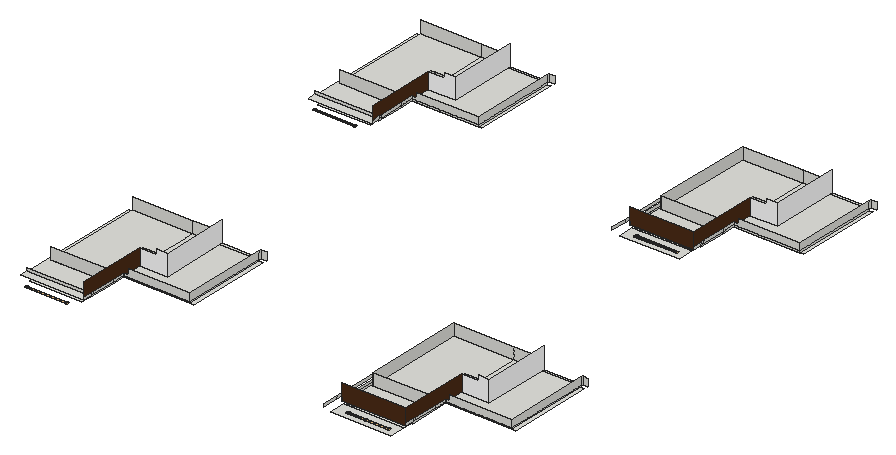
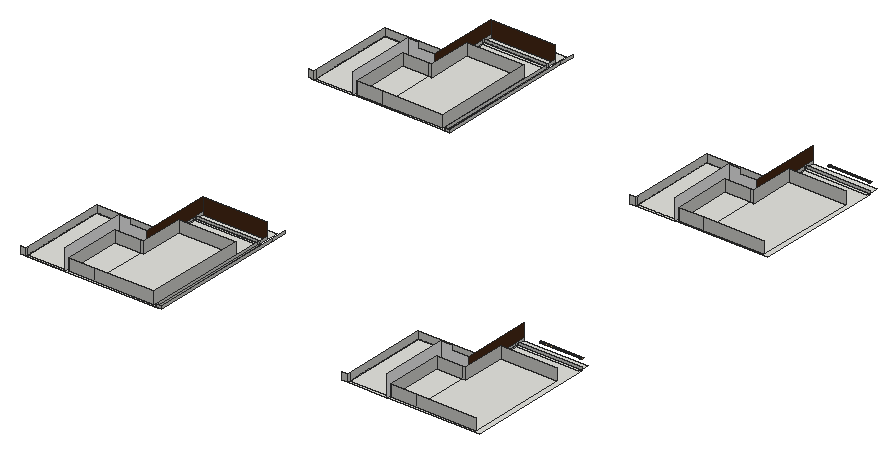
# SketchUp Ruby script. Lengths in inches.
U = 1.inch
M = Sketchup.active_model
def pt(a) = Geom::Point3d.new(a.map { |v| v * U })
def face(e, loops, mat)
  f = e.add_face(loops[0].map { |a| pt(a) })
  loops[1..].each { |l| e.add_face(l.map { |a| pt(a) }).erase! }
  f.material = f.back_material = mat if mat
  f
end
# faces: each face lists its corners as indices into pts; further lists are holes
def faces(e, pts, list, mat = nil) = list.each { |f| face(e, (f[0].is_a?(Array) ? f : [f]).map { |l| l.map { |i| pts[i] } }, mat) }
# xy, xz, yz: faces in a plane at the given z, y or x. An outline is a flat list of corners, or four numbers for a rectangle; further outlines are holes
def ring(l) = l.size == 4 ? [[l[0], l[1]], [l[2], l[1]], [l[2], l[3]], [l[0], l[3]]] : l.each_slice(2).to_a
def flat(e, list, mat, &to3) = list.each { |f| face(e, (f[0].is_a?(Array) ? f : [f]).map { |l| ring(l).map { |u, v| to3.(u, v) } }, mat) }
def xy(e, z, list, mat = nil) = flat(e, list, mat) { |x, y| [x, y, z] }
def xz(e, y, list, mat = nil) = flat(e, list, mat) { |x, z| [x, y, z] }
def yz(e, x, list, mat = nil) = flat(e, list, mat) { |y, z| [x, y, z] }
def lines(e, pts, list) = list.each { |a, b| e.add_line(pt(pts[a]), pt(pts[b])) }
# prism: a flat outline (further loops are holes) pulled along v
def prism(e, loops, v, mat = nil)
  f = face(e, loops, mat); d = Geom::Vector3d.new(v.map { |x| x * U })
  f.pushpull(f.normal.samedirection?(d) ? d.length : -d.length)
end
def box(e, o, s, mat = nil) = prism(e, [[o, [o[0] + s[0], o[1], o[2]], [o[0] + s[0], o[1] + s[1], o[2]], [o[0], o[1] + s[1], o[2]]]], [0, 0, s[2]], mat)
def at(x, y, z, deg = 0) = Geom::Transformation.translation(pt([x, y, z])) * Geom::Transformation.rotation(ORIGIN, Z_AXIS, deg.degrees)
def axes(o, x, y, z) = Geom::Transformation.new([*x, 0, *y, 0, *z, 0, *pt(o).to_a, 1])
def part(name) = M.definitions.add(name)
# library, detail: a bought-in or finely detailed component or shape, given as its bounding box
def library(name, o, s) = part(name).tap { |d| box(d.entities, o, s) }
def detail(e, o, s) = box(e.add_group.entities, o, s)
def put(e, d, t, mat = nil) = e.add_instance(d, t).tap { |i| i.material = mat if mat }
def group(e, t, mat = nil) = e.add_group.tap { |g| g.transformation = t; g.material = mat if mat }.entities
root = M.entities
M.materials.add("[Color M00]").color = [255, 255, 255]
M.materials.add("[Wood Veneer 01]").color = [76, 44, 23]
c1 = library("Group\#25",[-0.5,-0.5,-0.05],[119,6.375,0.22])
xy(root,257.1875,[[[2977.35,592.75,3143.91,636.6875],[3008.92,609.37,3009.62,609.46,3010.27,609.73,3010.82,610.15,3011.25,610.71,3011.52,611.36,3011.61,612.06,3011.52,612.75,3011.25,613.4,3010.82,613.96,3010.27,614.38,3009.62,614.65,3008.92,614.74,3008.23,614.65,3007.58,614.38,3007.02,613.96,3006.6,613.4,3006.33,612.75,3006.24,612.06,3006.33,611.36,3006.6,610.71,3007.02,610.15,3007.58,609.73,3008.23,609.46],[3056.92,609.37,3057.62,609.46,3058.27,609.73,3058.82,610.15,3059.25,610.71,3059.52,611.36,3059.61,612.06,3059.52,612.75,3059.25,613.4,3058.82,613.96,3058.27,614.38,3057.62,614.65,3056.92,614.74,3056.23,614.65,3055.58,614.38,3055.02,613.96,3054.6,613.4,3054.33,612.75,3054.24,612.06,3054.33,611.36,3054.6,610.71,3055.02,610.15,3055.58,609.73,3056.23,609.46],[3121.55,609.37,3122.24,609.46,3122.89,609.73,3123.45,610.15,3123.875,610.71,3124.14,611.36,3124.24,612.06,3124.14,612.75,3123.875,613.4,3123.45,613.96,3122.89,614.38,3122.24,614.65,3121.55,614.74,3120.85,614.65,3120.2,614.38,3119.65,613.96,3119.22,613.4,3118.95,612.75,3118.86,612.06,3118.95,611.36,3119.22,610.71,3119.65,610.15,3120.2,609.73,3120.85,609.46]],[2106.51,636.6875,2251.32,660.21],[2986.73,636.6875,2999.1,660.21],[2999.1,636.6875,3143.91,660.21],[[2977.35,1592.1,3143.91,1636.04],[3008.92,1608.72,3009.62,1608.8125,3010.27,1609.08,3010.82,1609.51,3011.25,1610.07,3011.52,1610.71,3011.61,1611.41,3011.52,1612.11,3011.25,1612.75,3010.82,1613.3125,3010.27,1613.74,3009.62,1614.01,3008.92,1614.1,3008.23,1614.01,3007.58,1613.74,3007.02,1613.3125,3006.6,1612.75,3006.33,1612.11,3006.24,1611.41,3006.33,1610.71,3006.6,1610.07,3007.02,1609.51,3007.58,1609.08,3008.23,1608.8125],[3056.92,1608.72,3057.62,1608.8125,3058.27,1609.08,3058.82,1609.51,3059.25,1610.07,3059.52,1610.71,3059.61,1611.41,3059.52,1612.11,3059.25,1612.75,3058.82,1613.3125,3058.27,1613.74,3057.62,1614.01,3056.92,1614.1,3056.23,1614.01,3055.58,1613.74,3055.02,1613.3125,3054.6,1612.75,3054.33,1612.11,3054.24,1611.41,3054.33,1610.71,3054.6,1610.07,3055.02,1609.51,3055.58,1609.08,3056.23,1608.8125],[3121.55,1608.72,3122.24,1608.8125,3122.89,1609.08,3123.45,1609.51,3123.875,1610.07,3124.14,1610.71,3124.24,1611.41,3124.14,1612.11,3123.875,1612.75,3123.45,1613.3125,3122.89,1613.74,3122.24,1614.01,3121.55,1614.1,3120.85,1614.01,3120.2,1613.74,3119.65,1613.3125,3119.22,1612.75,3118.95,1612.11,3118.86,1611.41,3118.95,1610.71,3119.22,1610.07,3119.65,1609.51,3120.2,1609.08,3120.85,1608.8125]],
  [2106.51,1636.04,2251.32,1659.57],[2986.73,1636.04,2999.1,1659.57],[2999.1,1636.04,3143.91,1659.57]])
xy(root,259.3125,[[2079.65,660.21,2079.65,1012.63,2440.84,1012.63,2440.84,774.3125,2256.86,774.3125,2256.86,660.21],[2972.24,660.21,2972.24,1012.63,3333.43,1012.63,3333.43,774.3125,3149.44,774.3125,3149.44,660.21],[2440.84,774.3125,2450.84,1012.63],[3333.43,774.3125,3343.43,1012.63],[2079.65,1659.57,2079.65,2011.98,2440.84,2011.98,2440.84,1773.67,2256.86,1773.67,2256.86,1659.57],
  [2972.24,1659.57,2972.24,2011.98,3333.43,2011.98,3333.43,1773.67,3149.44,1773.67,3149.44,1659.57],[2440.84,1773.67,2450.84,2011.98],[3333.43,1773.67,3343.43,2011.98]])
xy(root,262.875,[[2079.65,636.86,2256.86,660.21],[2972.24,636.86,3149.44,660.21],[2079.65,660.21,2256.86,668.18],[2972.24,660.21,3149.44,668.18],[2089.96,731.45,2247.33,731.45,2247.33,852.1875,2256.86,852.1875,2256.86,1012.63,2089.96,1012.63],
  [2982.55,731.45,3139.92,731.45,3139.92,852.1875,3149.44,852.1875,3149.44,1012.63,2982.55,1012.63],[2256.86,774.3125,2440.84,774.3125,2440.84,1012.63,2333.29,1012.63,2333.29,829.8125,2256.86,829.8125],[3149.44,774.3125,3333.43,774.3125,3333.43,1012.63,3225.88,1012.63,3225.88,829.8125,3149.44,829.8125],[2256.86,852.1875,2327.29,1012.63],[3149.44,852.1875,3219.88,1012.63],
  [2333.29,1012.63,2440.84,1019],[3225.88,1012.63,3333.43,1019],[2079.65,1636.22,2256.86,1659.57],[2972.24,1636.22,3149.44,1659.57],[2079.65,1659.57,2256.86,1667.53],
  [2972.24,1659.57,3149.44,1667.53],[2089.96,1730.8,2247.33,1730.8,2247.33,1851.54,2256.86,1851.54,2256.86,2011.98,2089.96,2011.98],[2982.55,1730.8,3139.92,1730.8,3139.92,1851.54,3149.44,1851.54,3149.44,2011.98,2982.55,2011.98],[2256.86,1773.67,2440.84,1773.67,2440.84,2011.98,2333.29,2011.98,2333.29,1829.17,2256.86,1829.17],[3149.44,1773.67,3333.43,1773.67,3333.43,2011.98,3225.88,2011.98,3225.88,1829.17,3149.44,1829.17],
  [2256.86,1851.54,2327.29,2011.98],[3149.44,1851.54,3219.88,2011.98],[2333.29,2011.98,2440.84,2018.36],[3225.88,2011.98,3333.43,2018.36]])
xz(root,636.86,[[2972.24,262.875,3149.44,307.5]],"[Wood Veneer 01]")
xz(root,660.21,[[2972.24,259.3125,3149.44,262.875],[2079.65,262.875,2256.86,270.375],[2972.24,262.875,3149.44,270.375]])
xz(root,731.45,[[2089.96,262.875,2247.33,295.8125],[2982.55,262.875,3139.92,295.8125]])
xz(root,774.3125,[[2256.86,259.3125,2440.84,262.875],[3149.44,259.3125,3333.43,262.875],[2256.86,262.875,2256.86,270.375,2269.48,270.375,2269.48,283.9375,2440.84,283.9375,2440.84,262.875],[3149.44,262.875,3149.44,270.375,3162.07,270.375,3162.07,283.9375,3333.43,283.9375,3333.43,262.875]])
xz(root,829.8125,[[2256.86,262.875,2333.29,262.875,2333.29,320.75,2303.29,320.75,2303.29,307.5,2256.86,307.5],[3149.44,262.875,3225.88,262.875,3225.88,320.75,3195.88,320.75,3195.88,307.5,3149.44,307.5]],"[Color M00]")
xz(root,852.1875,[[2247.33,262.875,2256.86,295.8125],[2256.86,262.875,2327.29,295.8125],[3139.92,262.875,3149.44,295.8125],[3149.44,262.875,3219.88,295.8125]])
xz(root,1012.63,[[2089.96,262.875,2256.86,295.8125],[2256.86,262.875,2327.29,295.8125],[2982.55,262.875,3149.44,295.8125],[3149.44,262.875,3219.88,295.8125]])
xz(root,1019,[[2440.84,262.875,2456.54,283.9375],[2957.51,262.875,2972.24,270.375],[3333.43,262.875,3349.13,283.9375]])
xz(root,1636.22,[[2972.24,262.875,3149.44,307.5]],"[Wood Veneer 01]")
xz(root,1659.57,[[2972.24,259.3125,3149.44,262.875],[2079.65,262.875,2256.86,270.375],[2972.24,262.875,3149.44,270.375]])
xz(root,1730.8,[[2089.96,262.875,2247.33,295.8125],[2982.55,262.875,3139.92,295.8125]])
xz(root,1773.67,[[2256.86,259.3125,2440.84,262.875],[3149.44,259.3125,3333.43,262.875],[2256.86,262.875,2256.86,270.375,2269.48,270.375,2269.48,283.9375,2440.84,283.9375,2440.84,262.875],[3149.44,262.875,3149.44,270.375,3162.07,270.375,3162.07,283.9375,3333.43,283.9375,3333.43,262.875]])
xz(root,1829.17,[[2256.86,262.875,2333.29,262.875,2333.29,320.75,2303.29,320.75,2303.29,307.5,2256.86,307.5],[3149.44,262.875,3225.88,262.875,3225.88,320.75,3195.88,320.75,3195.88,307.5,3149.44,307.5]],"[Color M00]")
xz(root,1851.54,[[2247.33,262.875,2256.86,295.8125],[2256.86,262.875,2327.29,295.8125],[3139.92,262.875,3149.44,295.8125],[3149.44,262.875,3219.88,295.8125]])
xz(root,2011.98,[[2089.96,262.875,2256.86,295.8125],[2256.86,262.875,2327.29,295.8125],[2982.55,262.875,3149.44,295.8125],[3149.44,262.875,3219.88,295.8125]])
xz(root,2018.36,[[2440.84,262.875,2456.54,283.9375],[2957.51,262.875,2972.24,270.375],[3333.43,262.875,3349.13,283.9375]])
yz(root,2247.33,[[731.45,262.875,852.1875,295.8125],[1730.8,262.875,1851.54,295.8125]])
yz(root,2256.86,[[660.21,259.3125,735.75,262.875],[735.75,259.3125,774.3125,262.875],[1659.57,259.3125,1735.1,262.875],[1735.1,259.3125,1773.67,262.875],[636.86,262.875,660.21,270.375],
  [660.21,262.875,668.18,270.375],[668.18,262.875,735.75,270.375],[735.75,262.875,774.3125,270.375],[1636.22,262.875,1659.57,270.375],[1659.57,262.875,1667.53,270.375],
  [1667.53,262.875,1735.1,270.375],[1735.1,262.875,1773.67,270.375]])
yz(root,2256.86,[[774.3125,262.875,829.8125,262.875,829.8125,307.5,636.86,307.5,636.86,270.375,774.3125,270.375],[1773.67,262.875,1829.17,262.875,1829.17,307.5,1636.22,307.5,1636.22,270.375,1773.67,270.375]],"[Wood Veneer 01]")
yz(root,2327.29,[[852.1875,262.875,1012.63,295.8125],[1851.54,262.875,2011.98,295.8125]])
yz(root,2333.29,[[829.8125,262.875,1019,320.75],[1829.17,262.875,2018.36,320.75]],"[Color M00]")
yz(root,2440.84,[[774.3125,259.3125,1012.63,262.875],[1773.67,259.3125,2011.98,262.875],[774.3125,262.875,1012.63,283.9375],[1012.63,262.875,1019,283.9375],[1773.67,262.875,2011.98,283.9375],
  [2011.98,262.875,2018.36,283.9375]])
yz(root,2957.51,[[592.75,262.875,636.6875,270.375],[636.6875,262.875,1019,270.375],[1592.1,262.875,1636.04,270.375],[1636.04,262.875,2018.36,270.375]])
yz(root,2972.24,[[660.21,259.3125,1012.63,262.875],[1659.57,259.3125,2011.98,262.875],[636.86,262.875,660.21,270.375],[660.21,262.875,668.18,270.375],[668.18,262.875,1012.63,270.375],
  [1012.63,262.875,1019,270.375],[1636.22,262.875,1659.57,270.375],[1659.57,262.875,1667.53,270.375],[1667.53,262.875,2011.98,270.375],[2011.98,262.875,2018.36,270.375]])
yz(root,2982.55,[[731.45,262.875,1012.63,295.8125],[1730.8,262.875,2011.98,295.8125]])
yz(root,3139.92,[[731.45,262.875,852.1875,295.8125],[1730.8,262.875,1851.54,295.8125]])
yz(root,3149.44,[[660.21,259.3125,735.75,262.875],[735.75,259.3125,774.3125,262.875],[1659.57,259.3125,1735.1,262.875],[1735.1,259.3125,1773.67,262.875],[636.86,262.875,660.21,270.375],
  [660.21,262.875,668.18,270.375],[668.18,262.875,735.75,270.375],[735.75,262.875,774.3125,270.375],[1636.22,262.875,1659.57,270.375],[1659.57,262.875,1667.53,270.375],
  [1667.53,262.875,1735.1,270.375],[1735.1,262.875,1773.67,270.375]])
yz(root,3149.44,[[774.3125,262.875,829.8125,262.875,829.8125,307.5,636.86,307.5,636.86,270.375,774.3125,270.375],[1773.67,262.875,1829.17,262.875,1829.17,307.5,1636.22,307.5,1636.22,270.375,1773.67,270.375]],"[Wood Veneer 01]")
yz(root,3219.88,[[852.1875,262.875,1012.63,295.8125],[1851.54,262.875,2011.98,295.8125]])
yz(root,3225.88,[[829.8125,262.875,1019,320.75],[1829.17,262.875,2018.36,320.75]],"[Color M00]")
yz(root,3333.43,[[774.3125,259.3125,1012.63,262.875],[1773.67,259.3125,2011.98,262.875],[774.3125,262.875,1012.63,283.9375],[1012.63,262.875,1019,283.9375],[1773.67,262.875,2011.98,283.9375],
  [2011.98,262.875,2018.36,283.9375]])
p = [[2228.96,609.37,257.1875],[2228.26,609.46,257.1875],[2228.26,609.46,257.8125],[2228.96,609.37,257.8125],[2229.65,609.46,257.1875],[2229.65,609.46,257.8125],
  [3008.92,609.37,257.1875],[3008.23,609.46,257.1875],[3008.23,609.46,257.6875],[3008.92,609.37,257.6875],[3009.62,609.46,257.1875],[3009.62,609.46,257.6875],
  [3056.92,609.37,257.1875],[3056.23,609.46,257.1875],[3056.23,609.46,257.8125],[3056.92,609.37,257.8125],[3057.62,609.46,257.1875],[3057.62,609.46,257.8125],
  [3121.55,609.37,257.1875],[3120.85,609.46,257.1875],[3120.85,609.46,257.8125],[3121.55,609.37,257.8125],[3122.24,609.46,257.1875],[3122.24,609.46,257.8125],
  [2227.61,609.73,257.1875],[2227.61,609.73,257.8125],[2230.3,609.73,257.1875],[2230.3,609.73,257.8125],[3007.58,609.73,257.1875],[3007.58,609.73,257.6875],
  [3010.27,609.73,257.1875],[3010.27,609.73,257.6875],[3055.58,609.73,257.1875],[3055.58,609.73,257.8125],[3058.27,609.73,257.1875],[3058.27,609.73,257.8125],
  [3120.2,609.73,257.1875],[3120.2,609.73,257.8125],[3122.89,609.73,257.1875],[3122.89,609.73,257.8125],[2227.06,610.15,257.1875],[2227.06,610.15,257.8125],
  [2230.86,610.15,257.1875],[2230.86,610.15,257.8125],[3007.02,610.15,257.1875],[3007.02,610.15,257.6875],[3010.82,610.15,257.1875],[3010.82,610.15,257.6875],
  [3055.02,610.15,257.1875],[3055.02,610.15,257.8125],[3058.82,610.15,257.1875],[3058.82,610.15,257.8125],[3119.65,610.15,257.1875],[3119.65,610.15,257.8125],
  [3123.45,610.15,257.1875],[3123.45,610.15,257.8125],[2226.63,610.71,257.1875],[2226.63,610.71,257.8125],[2231.29,610.71,257.1875],[2231.29,610.71,257.8125],
  [3006.6,610.71,257.1875],[3006.6,610.71,257.6875],[3011.25,610.71,257.1875],[3011.25,610.71,257.6875],[3054.6,610.71,257.1875],[3054.6,610.71,257.8125],
  [3059.25,610.71,257.1875],[3059.25,610.71,257.8125],[3119.22,610.71,257.1875],[3119.22,610.71,257.8125],[3123.875,610.71,257.1875],[3123.875,610.71,257.8125],
  [2226.36,611.36,257.1875],[2226.36,611.36,257.8125],[2231.55,611.36,257.1875],[2231.55,611.36,257.8125],[3006.33,611.36,257.1875],[3006.33,611.36,257.6875],
  [3011.52,611.36,257.1875],[3011.52,611.36,257.6875],[3054.33,611.36,257.1875],[3054.33,611.36,257.8125],[3059.52,611.36,257.1875],[3059.52,611.36,257.8125],
  [3118.95,611.36,257.1875],[3118.95,611.36,257.8125],[3124.14,611.36,257.1875],[3124.14,611.36,257.8125],[2226.27,612.06,257.1875],[2226.27,612.06,257.8125],
  [2231.65,612.06,257.1875],[2231.65,612.06,257.8125],[3006.24,612.06,257.1875],[3006.24,612.06,257.6875],[3011.61,612.06,257.1875],[3011.61,612.06,257.6875],
  [3054.24,612.06,257.1875],[3054.24,612.06,257.8125],[3059.61,612.06,257.1875],[3059.61,612.06,257.8125],[3118.86,612.06,257.1875],[3118.86,612.06,257.8125],
  [3124.24,612.06,257.1875],[3124.24,612.06,257.8125],[2226.36,612.75,257.1875],[2226.36,612.75,257.8125],[2231.55,612.75,257.1875],[2231.55,612.75,257.8125],
  [3006.33,612.75,257.1875],[3006.33,612.75,257.6875],[3011.52,612.75,257.1875],[3011.52,612.75,257.6875],[3054.33,612.75,257.1875],[3054.33,612.75,257.8125],
  [3059.52,612.75,257.1875],[3059.52,612.75,257.8125],[3118.95,612.75,257.1875],[3118.95,612.75,257.8125],[3124.14,612.75,257.1875],[3124.14,612.75,257.8125],
  [2226.63,613.4,257.1875],[2226.63,613.4,257.8125],[2231.29,613.4,257.1875],[2231.29,613.4,257.8125],[3006.6,613.4,257.1875],[3006.6,613.4,257.6875],
  [3011.25,613.4,257.1875],[3011.25,613.4,257.6875],[3054.6,613.4,257.1875],[3054.6,613.4,257.8125],[3059.25,613.4,257.1875],[3059.25,613.4,257.8125],
  [3119.22,613.4,257.1875],[3119.22,613.4,257.8125],[3123.875,613.4,257.1875],[3123.875,613.4,257.8125],[2227.06,613.96,257.1875],[2227.06,613.96,257.8125],
  [2230.86,613.96,257.1875],[2230.86,613.96,257.8125],[3007.02,613.96,257.1875],[3007.02,613.96,257.6875],[3010.82,613.96,257.1875],[3010.82,613.96,257.6875],
  [3055.02,613.96,257.1875],[3055.02,613.96,257.8125],[3058.82,613.96,257.1875],[3058.82,613.96,257.8125],[3119.65,613.96,257.1875],[3119.65,613.96,257.8125],
  [3123.45,613.96,257.1875],[3123.45,613.96,257.8125],[2227.61,614.38,257.1875],[2227.61,614.38,257.8125],[2230.3,614.38,257.1875],[2230.3,614.38,257.8125],
  [3007.58,614.38,257.1875],[3007.58,614.38,257.6875],[3010.27,614.38,257.1875],[3010.27,614.38,257.6875],[3055.58,614.38,257.1875],[3055.58,614.38,257.8125],
  [3058.27,614.38,257.1875],[3058.27,614.38,257.8125],[3120.2,614.38,257.1875],[3120.2,614.38,257.8125],[3122.89,614.38,257.1875],[3122.89,614.38,257.8125],
  [2228.26,614.65,257.1875],[2228.26,614.65,257.8125],[2229.65,614.65,257.1875],[2229.65,614.65,257.8125],[3008.23,614.65,257.1875],[3008.23,614.65,257.6875],
  [3009.62,614.65,257.1875],[3009.62,614.65,257.6875],[3056.23,614.65,257.1875],[3056.23,614.65,257.8125],[3057.62,614.65,257.1875],[3057.62,614.65,257.8125],
  [3120.85,614.65,257.1875],[3120.85,614.65,257.8125],[3122.24,614.65,257.1875],[3122.24,614.65,257.8125],[2228.96,614.74,257.1875],[2228.96,614.74,257.8125],
  [3008.92,614.74,257.1875],[3008.92,614.74,257.6875],[3056.92,614.74,257.1875],[3056.92,614.74,257.8125],[3121.55,614.74,257.1875],[3121.55,614.74,257.8125],
  [2228.96,1608.72,257.1875],[2228.26,1608.8125,257.1875],[2228.26,1608.8125,257.8125],[2228.96,1608.72,257.8125],[2229.65,1608.8125,257.1875],[2229.65,1608.8125,257.8125],
  [3008.92,1608.72,257.1875],[3008.23,1608.8125,257.1875],[3008.23,1608.8125,257.6875],[3008.92,1608.72,257.6875],[3009.62,1608.8125,257.1875],[3009.62,1608.8125,257.6875],
  [3056.92,1608.72,257.1875],[3056.23,1608.8125,257.1875],[3056.23,1608.8125,257.8125],[3056.92,1608.72,257.8125],[3057.62,1608.8125,257.1875],[3057.62,1608.8125,257.8125],
  [3121.55,1608.72,257.1875],[3120.85,1608.8125,257.1875],[3120.85,1608.8125,257.8125],[3121.55,1608.72,257.8125],[3122.24,1608.8125,257.1875],[3122.24,1608.8125,257.8125],
  [2227.61,1609.08,257.1875],[2227.61,1609.08,257.8125],[2230.3,1609.08,257.1875],[2230.3,1609.08,257.8125],[3007.58,1609.08,257.1875],[3007.58,1609.08,257.6875],
  [3010.27,1609.08,257.1875],[3010.27,1609.08,257.6875],[3055.58,1609.08,257.1875],[3055.58,1609.08,257.8125],[3058.27,1609.08,257.1875],[3058.27,1609.08,257.8125],
  [3120.2,1609.08,257.1875],[3120.2,1609.08,257.8125],[3122.89,1609.08,257.1875],[3122.89,1609.08,257.8125],[2227.06,1609.51,257.1875],[2227.06,1609.51,257.8125],
  [2230.86,1609.51,257.1875],[2230.86,1609.51,257.8125],[3007.02,1609.51,257.1875],[3007.02,1609.51,257.6875],[3010.82,1609.51,257.1875],[3010.82,1609.51,257.6875],
  [3055.02,1609.51,257.1875],[3055.02,1609.51,257.8125],[3058.82,1609.51,257.1875],[3058.82,1609.51,257.8125],[3119.65,1609.51,257.1875],[3119.65,1609.51,257.8125],
  [3123.45,1609.51,257.1875],[3123.45,1609.51,257.8125],[2226.63,1610.07,257.1875],[2226.63,1610.07,257.8125],[2231.29,1610.07,257.1875],[2231.29,1610.07,257.8125],
  [3006.6,1610.07,257.1875],[3006.6,1610.07,257.6875],[3011.25,1610.07,257.1875],[3011.25,1610.07,257.6875],[3054.6,1610.07,257.1875],[3054.6,1610.07,257.8125],
  [3059.25,1610.07,257.1875],[3059.25,1610.07,257.8125],[3119.22,1610.07,257.1875],[3119.22,1610.07,257.8125],[3123.875,1610.07,257.1875],[3123.875,1610.07,257.8125],
  [2226.36,1610.71,257.1875],[2226.36,1610.71,257.8125],[2231.55,1610.71,257.1875],[2231.55,1610.71,257.8125],[3006.33,1610.71,257.1875],[3006.33,1610.71,257.6875],
  [3011.52,1610.71,257.1875],[3011.52,1610.71,257.6875],[3054.33,1610.71,257.1875],[3054.33,1610.71,257.8125],[3059.52,1610.71,257.1875],[3059.52,1610.71,257.8125],
  [3118.95,1610.71,257.1875],[3118.95,1610.71,257.8125],[3124.14,1610.71,257.1875],[3124.14,1610.71,257.8125],[2226.27,1611.41,257.1875],[2226.27,1611.41,257.8125],
  [2231.65,1611.41,257.1875],[2231.65,1611.41,257.8125],[3006.24,1611.41,257.1875],[3006.24,1611.41,257.6875],[3011.61,1611.41,257.1875],[3011.61,1611.41,257.6875],
  [3054.24,1611.41,257.1875],[3054.24,1611.41,257.8125],[3059.61,1611.41,257.1875],[3059.61,1611.41,257.8125],[3118.86,1611.41,257.1875],[3118.86,1611.41,257.8125],
  [3124.24,1611.41,257.1875],[3124.24,1611.41,257.8125],[2226.36,1612.11,257.1875],[2226.36,1612.11,257.8125],[2231.55,1612.11,257.1875],[2231.55,1612.11,257.8125],
  [3006.33,1612.11,257.1875],[3006.33,1612.11,257.6875],[3011.52,1612.11,257.1875],[3011.52,1612.11,257.6875],[3054.33,1612.11,257.1875],[3054.33,1612.11,257.8125],
  [3059.52,1612.11,257.1875],[3059.52,1612.11,257.8125],[3118.95,1612.11,257.1875],[3118.95,1612.11,257.8125],[3124.14,1612.11,257.1875],[3124.14,1612.11,257.8125],
  [2226.63,1612.75,257.1875],[2226.63,1612.75,257.8125],[2231.29,1612.75,257.1875],[2231.29,1612.75,257.8125],[3006.6,1612.75,257.1875],[3006.6,1612.75,257.6875],
  [3011.25,1612.75,257.1875],[3011.25,1612.75,257.6875],[3054.6,1612.75,257.1875],[3054.6,1612.75,257.8125],[3059.25,1612.75,257.1875],[3059.25,1612.75,257.8125],
  [3119.22,1612.75,257.1875],[3119.22,1612.75,257.8125],[3123.875,1612.75,257.1875],[3123.875,1612.75,257.8125],[2227.06,1613.3125,257.1875],[2227.06,1613.3125,257.8125],
  [2230.86,1613.3125,257.1875],[2230.86,1613.3125,257.8125],[3007.02,1613.3125,257.1875],[3007.02,1613.3125,257.6875],[3010.82,1613.3125,257.1875],[3010.82,1613.3125,257.6875],
  [3055.02,1613.3125,257.1875],[3055.02,1613.3125,257.8125],[3058.82,1613.3125,257.1875],[3058.82,1613.3125,257.8125],[3119.65,1613.3125,257.1875],[3119.65,1613.3125,257.8125],
  [3123.45,1613.3125,257.1875],[3123.45,1613.3125,257.8125],[2227.61,1613.74,257.1875],[2227.61,1613.74,257.8125],[2230.3,1613.74,257.1875],[2230.3,1613.74,257.8125],
  [3007.58,1613.74,257.1875],[3007.58,1613.74,257.6875],[3010.27,1613.74,257.1875],[3010.27,1613.74,257.6875],[3055.58,1613.74,257.1875],[3055.58,1613.74,257.8125],
  [3058.27,1613.74,257.1875],[3058.27,1613.74,257.8125],[3120.2,1613.74,257.1875],[3120.2,1613.74,257.8125],[3122.89,1613.74,257.1875],[3122.89,1613.74,257.8125],
  [2228.26,1614.01,257.1875],[2228.26,1614.01,257.8125],[2229.65,1614.01,257.1875],[2229.65,1614.01,257.8125],[3008.23,1614.01,257.1875],[3008.23,1614.01,257.6875],
  [3009.62,1614.01,257.1875],[3009.62,1614.01,257.6875],[3056.23,1614.01,257.1875],[3056.23,1614.01,257.8125],[3057.62,1614.01,257.1875],[3057.62,1614.01,257.8125],
  [3120.85,1614.01,257.1875],[3120.85,1614.01,257.8125],[3122.24,1614.01,257.1875],[3122.24,1614.01,257.8125],[2228.96,1614.1,257.1875],[2228.96,1614.1,257.8125],
  [3008.92,1614.1,257.1875],[3008.92,1614.1,257.6875],[3056.92,1614.1,257.1875],[3056.92,1614.1,257.8125],[3121.55,1614.1,257.1875],[3121.55,1614.1,257.8125]]
faces(root,p,[[0,1,2,3],[4,0,3,5],[6,7,8,9],[10,6,9,11],[12,13,14,15],[16,12,15,17],[18,19,20,21],[22,18,21,23],
  [1,24,25,2],[26,4,5,27],[7,28,29,8],[30,10,11,31],[13,32,33,14],[34,16,17,35],[19,36,37,20],[38,22,23,39],
  [24,40,41,25],[42,26,27,43],[28,44,45,29],[46,30,31,47],[32,48,49,33],[50,34,35,51],[36,52,53,37],[54,38,39,55],
  [40,56,57,41],[58,42,43,59],[44,60,61,45],[62,46,47,63],[48,64,65,49],[66,50,51,67],[52,68,69,53],[70,54,55,71],
  [56,72,73,57],[74,58,59,75],[60,76,77,61],[78,62,63,79],[64,80,81,65],[82,66,67,83],[68,84,85,69],[86,70,71,87],
  [72,88,89,73],[90,74,75,91],[76,92,93,77],[94,78,79,95],[80,96,97,81],[98,82,83,99],[84,100,101,85],[102,86,87,103],
  [88,104,105,89],[106,90,91,107],[92,108,109,93],[110,94,95,111],[96,112,113,97],[114,98,99,115],[100,116,117,101],[118,102,103,119],
  [104,120,121,105],[122,106,107,123],[108,124,125,109],[126,110,111,127],[112,128,129,113],[130,114,115,131],[116,132,133,117],[134,118,119,135],
  [120,136,137,121],[138,122,123,139],[124,140,141,125],[142,126,127,143],[128,144,145,129],[146,130,131,147],[132,148,149,133],[150,134,135,151],
  [136,152,153,137],[154,138,139,155],[140,156,157,141],[158,142,143,159],[144,160,161,145],[162,146,147,163],[148,164,165,149],[166,150,151,167],
  [152,168,169,153],[170,154,155,171],[156,172,173,157],[174,158,159,175],[160,176,177,161],[178,162,163,179],[164,180,181,165],[182,166,167,183],
  [168,184,185,169],[184,170,171,185],[172,186,187,173],[186,174,175,187],[176,188,189,177],[188,178,179,189],[180,190,191,181],[190,182,183,191],
  [192,193,194,195],[196,192,195,197],[198,199,200,201],[202,198,201,203],[204,205,206,207],[208,204,207,209],[210,211,212,213],[214,210,213,215],
  [193,216,217,194],[218,196,197,219],[199,220,221,200],[222,202,203,223],[205,224,225,206],[226,208,209,227],[211,228,229,212],[230,214,215,231],
  [216,232,233,217],[234,218,219,235],[220,236,237,221],[238,222,223,239],[224,240,241,225],[242,226,227,243],[228,244,245,229],[246,230,231,247],
  [232,248,249,233],[250,234,235,251],[236,252,253,237],[254,238,239,255],[240,256,257,241],[258,242,243,259],[244,260,261,245],[262,246,247,263],
  [248,264,265,249],[266,250,251,267],[252,268,269,253],[270,254,255,271],[256,272,273,257],[274,258,259,275],[260,276,277,261],[278,262,263,279],
  [264,280,281,265],[282,266,267,283],[268,284,285,269],[286,270,271,287],[272,288,289,273],[290,274,275,291],[276,292,293,277],[294,278,279,295],
  [280,296,297,281],[298,282,283,299],[284,300,301,285],[302,286,287,303],[288,304,305,289],[306,290,291,307],[292,308,309,293],[310,294,295,311],
  [296,312,313,297],[314,298,299,315],[300,316,317,301],[318,302,303,319],[304,320,321,305],[322,306,307,323],[308,324,325,309],[326,310,311,327],
  [312,328,329,313],[330,314,315,331],[316,332,333,317],[334,318,319,335],[320,336,337,321],[338,322,323,339],[324,340,341,325],[342,326,327,343],
  [328,344,345,329],[346,330,331,347],[332,348,349,333],[350,334,335,351],[336,352,353,337],[354,338,339,355],[340,356,357,341],[358,342,343,359],
  [344,360,361,345],[362,346,347,363],[348,364,365,349],[366,350,351,367],[352,368,369,353],[370,354,355,371],[356,372,373,357],[374,358,359,375],
  [360,376,377,361],[376,362,363,377],[364,378,379,365],[378,366,367,379],[368,380,381,369],[380,370,371,381],[372,382,383,373],[382,374,375,383]])
put(root,c1,at(2113.65,1608.72,257.6875))
put(root,c1,at(2113.65,609.37,257.6875))
put(root,c1,at(3006.24,1608.72,257.6875))
put(root,c1,at(3006.24,609.37,257.6875))
